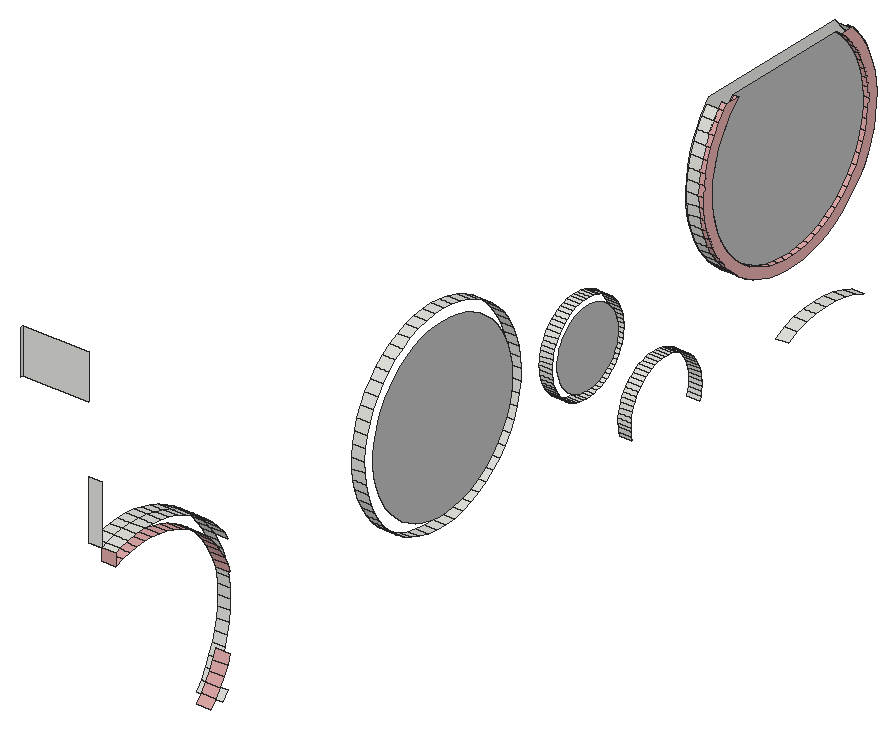
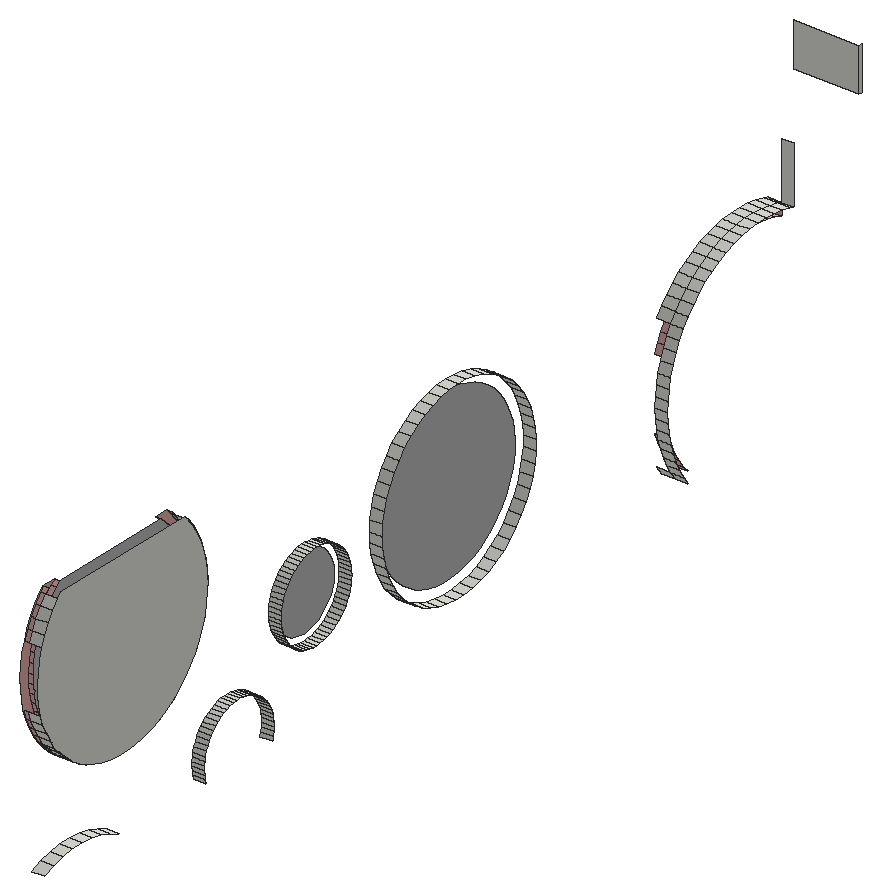
# SketchUp Ruby script. Lengths in inches.
U = 1.inch
M = Sketchup.active_model
def pt(a) = Geom::Point3d.new(a.map { |v| v * U })
def face(e, loops, mat)
  f = e.add_face(loops[0].map { |a| pt(a) })
  loops[1..].each { |l| e.add_face(l.map { |a| pt(a) }).erase! }
  f.material = f.back_material = mat if mat
  f
end
# faces: each face lists its corners as indices into pts; further lists are holes
def faces(e, pts, list, mat = nil) = list.each { |f| face(e, (f[0].is_a?(Array) ? f : [f]).map { |l| l.map { |i| pts[i] } }, mat) }
# xy, xz, yz: faces in a plane at the given z, y or x. An outline is a flat list of corners, or four numbers for a rectangle; further outlines are holes
def ring(l) = l.size == 4 ? [[l[0], l[1]], [l[2], l[1]], [l[2], l[3]], [l[0], l[3]]] : l.each_slice(2).to_a
def flat(e, list, mat, &to3) = list.each { |f| face(e, (f[0].is_a?(Array) ? f : [f]).map { |l| ring(l).map { |u, v| to3.(u, v) } }, mat) }
def xy(e, z, list, mat = nil) = flat(e, list, mat) { |x, y| [x, y, z] }
def xz(e, y, list, mat = nil) = flat(e, list, mat) { |x, z| [x, y, z] }
def yz(e, x, list, mat = nil) = flat(e, list, mat) { |y, z| [x, y, z] }
def lines(e, pts, list) = list.each { |a, b| e.add_line(pt(pts[a]), pt(pts[b])) }
# prism: a flat outline (further loops are holes) pulled along v
def prism(e, loops, v, mat = nil)
  f = face(e, loops, mat); d = Geom::Vector3d.new(v.map { |x| x * U })
  f.pushpull(f.normal.samedirection?(d) ? d.length : -d.length)
end
def box(e, o, s, mat = nil) = prism(e, [[o, [o[0] + s[0], o[1], o[2]], [o[0] + s[0], o[1] + s[1], o[2]], [o[0], o[1] + s[1], o[2]]]], [0, 0, s[2]], mat)
def at(x, y, z, deg = 0) = Geom::Transformation.translation(pt([x, y, z])) * Geom::Transformation.rotation(ORIGIN, Z_AXIS, deg.degrees)
def axes(o, x, y, z) = Geom::Transformation.new([*x, 0, *y, 0, *z, 0, *pt(o).to_a, 1])
def part(name) = M.definitions.add(name)
# library, detail: a bought-in or finely detailed component or shape, given as its bounding box
def library(name, o, s) = part(name).tap { |d| box(d.entities, o, s) }
def detail(e, o, s) = box(e.add_group.entities, o, s)
def put(e, d, t, mat = nil) = e.add_instance(d, t).tap { |i| i.material = mat if mat }
def group(e, t, mat = nil) = e.add_group.tap { |g| g.transformation = t; g.material = mat if mat }.entities
root = M.entities
M.materials.add("Generic").color = [224, 169, 169]
M.materials.add("[Mirror 01]").color = [185, 185, 185]
xy(root,95.3,[[9,116.01,10.6875,117.43]])
xy(root,95.3,[[10.6875,116.01,11.4375,117.43]],"Generic")
xy(root,96.65,[[10.6875,116.08,11.4375,117.37]],"Generic")
xz(root,0.4375,[[9,112.04,10.6875,120],[0,129.25,9,135.25]])
xz(root,0.4375,[[10.6875,110.34,12.625,112.04]],"Generic")
xz(root,89.3,[[9,99.77,10.6875,100.36]])
xz(root,102.58,[[9,86.91,10.6875,87.49]])
yz(root,0,[[0,129.25,0.4375,135.25]])
yz(root,9,[[116.01,95.3,117.43,95.3,118.85,95.43,120.24,95.71,121.6,96.11,122.91,96.65,124.17,97.31,125.36,98.09,126.46,98.97,127.48,99.97,128.4,101.05,129.2,102.22,129.89,103.46,130.46,104.76,130.9,106.11,131.2,107.5,131.375,108.91,131.41,110.32,131.31,111.74,131.07,113.14,130.69,114.51,130.19,115.84,129.5625,117.11,128.8125,118.3125,127.95,119.44,127.43,120,106.01,120,105.5,119.44,104.63,118.3125,103.89,117.11,103.26,115.84,102.75,114.51,102.38,113.14,102.14,111.74,102.04,110.32,102.07,108.91,102.24,107.5,102.55,106.11,102.99,104.76,103.56,103.46,104.25,102.22,105.05,101.05,105.97,99.97,106.98,98.97,108.09,98.09,109.28,97.31,110.53,96.65,111.85,96.11,113.21,95.71,114.6,95.43]])
yz(root,10.6875,[[59,90.55,60.3,90.67,61.57,90.94,62.81,91.35,63.99,91.89,65.11,92.55,66.15,93.34,67.09,94.23,67.93,95.23,68.66,96.31,69.26,97.46,69.73,98.67,70.07,99.93,70.27,101.22,70.32,102.52,70.23,103.81,70,105.1,69.625,106.34,69.12,107.54,68.48,108.68,67.73,109.74,66.86,110.7,65.89,111.57,64.83,112.33,63.69,112.96,62.49,113.47,61.25,113.84,59.96,114.07,58.67,114.16,57.37,114.11,56.08,113.91,54.82,113.57,53.61,113.1,52.46,112.49,51.38,111.77,50.39,110.93,49.49,109.98,48.71,108.94,48.04,107.82,47.5,106.64,47.1,105.4,46.83,104.13,46.71,102.83,46.72,101.53,46.89,100.24,47.1875,98.97,47.63,97.75,48.2,96.58,48.9,95.48,49.71,94.47,50.63,93.55,51.65,92.73,52.75,92.04,53.92,91.47,55.14,91.03,56.41,90.72,57.7,90.5625],[83.1,94.84,83.6,94.86,84.1,94.92,84.59,95.03,85.07,95.19,85.52,95.39,85.96,95.64,86.37,95.93,86.75,96.25,87.1,96.61,87.41,97.01,87.69,97.43,87.92,97.87,88.1,98.34,88.24,98.82,88.34,99.31,88.38,99.81,88.38,100.3125,88.33,100.81,88.23,101.3,88.08,101.78,87.89,102.24,87.66,102.6875,87.38,103.1,87.0625,103.49,86.71,103.85,86.33,104.17,85.91,104.45,85.47,104.69,85.01,104.89,84.53,105.04,84.04,105.15,83.55,105.21,83.04,105.22,82.55,105.18,82.05,105.09,81.57,104.96,81.1,104.78,80.65,104.55,80.23,104.28,79.83,103.98,79.47,103.63,79.14,103.26,78.84,102.85,78.59,102.42,78.38,101.96,78.22,101.49,78.1,101,78.03,100.5,78.01,100,78.04,99.5,78.11,99.01,78.24,98.52,78.41,98.05,78.62,97.6,78.875,97.16,79.17,96.76,79.51,96.39,79.875,96.05,80.28,95.75,80.7,95.48,81.15,95.26,81.625,95.09,82.11,94.96,82.6,94.88],[116.08,96.65,117.37,96.65,118.65,96.78,119.91,97.03,121.15,97.39,122.34,97.88,123.48,98.48,124.56,99.18,125.5625,99.99,126.49,100.89,127.32,101.875,128.05,102.9375,128.67,104.0625,129.1875,105.24,129.59,106.47,129.86,107.73,130.02,109,130.05,110.29,129.96,111.58,129.74,112.85,129.4,114.09,128.94,115.29,128.375,116.45,127.69,117.54,126.91,118.57,126.04,119.51,125.48,120,107.97,120,107.41,119.51,106.53,118.57,105.75,117.54,105.07,116.45,104.5,115.29,104.04,114.09,103.71,112.85,103.49,111.58,103.4,110.29,103.43,109,103.58,107.73,103.86,106.47,104.26,105.24,104.77,104.0625,105.4,102.94,106.13,101.875,106.96,100.89,107.88,99.99,108.89,99.18,109.97,98.48,111.11,97.88,112.3,97.39,113.53,97.03,114.8,96.78]],"[Mirror 01]")
yz(root,11.4375,[[116.01,95.3,117.43,95.3,118.85,95.43,120.24,95.71,121.6,96.11,122.91,96.65,124.17,97.31,125.36,98.09,126.46,98.97,127.48,99.97,128.4,101.05,129.2,102.22,129.89,103.46,130.46,104.76,130.9,106.11,131.2,107.5,131.375,108.91,131.41,110.32,131.31,111.74,131.07,113.14,130.69,114.51,130.19,115.84,129.5625,117.11,128.8125,118.3125,127.95,119.44,127.43,120,125.48,120,126.04,119.51,126.91,118.57,127.69,117.54,128.375,116.45,128.94,115.29,129.4,114.09,129.74,112.85,129.96,111.58,130.05,110.29,130.02,109,129.86,107.73,129.59,106.47,129.1875,105.24,128.67,104.0625,128.05,102.9375,127.32,101.875,126.49,100.89,125.5625,99.99,124.56,99.18,123.48,98.48,122.34,97.88,121.15,97.39,119.91,97.03,118.65,96.78,117.37,96.65,116.08,96.65,114.8,96.78,113.53,97.03,112.3,97.39,111.11,97.88,109.97,98.48,108.89,99.18,107.88,99.99,106.96,100.89,106.13,101.875,105.4,102.94,104.77,104.0625,104.26,105.24,103.86,106.47,103.58,107.73,103.43,109,103.4,110.29,103.49,111.58,103.71,112.85,104.04,114.09,104.5,115.29,105.07,116.45,105.75,117.54,106.53,118.57,107.41,119.51,107.97,120,106.01,120,105.5,119.44,104.63,118.3125,103.89,117.11,103.26,115.84,102.75,114.51,102.38,113.14,102.14,111.74,102.04,110.32,102.07,108.91,102.24,107.5,102.55,106.11,102.99,104.76,103.56,103.46,104.25,102.22,105.05,101.05,105.97,99.97,106.98,98.97,108.09,98.09,109.28,97.31,110.53,96.65,111.85,96.11,113.21,95.71,114.6,95.43]],"Generic")
p = [[10.6875,102.25,85.2],[10.6875,102.42,85.76],[9,102.42,85.76],[9,102.25,85.2],[10.6875,90.64,85.98],[10.6875,90.78,85.41],
  [9,90.78,85.41],[9,90.64,85.98],[10.6875,118.89,86.29],[10.6875,117.37,85.6],[9,117.37,85.6],[9,118.89,86.29],
  [10.6875,17.5,86.78],[10.6875,16.67,85.82],[12.625,16.67,85.82],[12.625,17.5,86.78],[10.6875,18.75,85.78],[10.6875,19.58,86.91],
  [9,19.58,86.91],[9,18.75,85.78],[12.625,19.58,86.91],[12.625,18.75,85.78],[10.6875,102.53,86.33],[9,102.53,86.33],
  [10.6875,90.55,86.55],[9,90.55,86.55],[10.6875,130.28,85.99],[10.6875,128.72,86.59],[9,128.72,86.59],[9,130.28,85.99],
  [10.6875,102.58,86.91],[9,102.58,86.91],[10.6875,120.48,86.8125],[9,120.48,86.8125],[10.6875,90.52,87.13],[9,90.52,87.13],
  [10.6875,127.1,87.01],[9,127.1,87.01],[10.6875,18.24,87.8],[12.625,18.24,87.8],[10.6875,122.11,87.15],[9,122.11,87.15],
  [10.6875,20.3,88.11],[9,20.3,88.11],[10.6875,125.45,87.25],[9,125.45,87.25],[10.6875,90.54,87.72],[9,90.54,87.72],
  [10.6875,123.78,87.29],[9,123.78,87.29],[10.6875,102.58,87.49],[10.6875,102.52,88.07],[9,102.52,88.07],[9,102.58,87.49],
  [10.6875,90.625,88.29],[9,90.625,88.29],[10.6875,18.9,88.88],[12.625,18.9,88.88],[10.6875,20.92,89.36],[9,20.92,89.36],
  [10.6875,102.4,88.64],[9,102.4,88.64],[10.6875,90.76,88.86],[9,90.76,88.86],[10.6875,102.23,89.2],[9,102.23,89.2],
  [10.6875,19.46,90.01],[12.625,19.46,90.01],[10.6875,90.95,89.41],[9,90.95,89.41],[10.6875,56.14,89.23],[10.6875,57.6,89.04],
  [9,57.6,89.04],[9,56.14,89.23],[10.6875,59.06,89.02],[9,59.06,89.02],[10.6875,60.53,89.17],[9,60.53,89.17],
  [10.6875,54.71,89.57],[9,54.71,89.57],[10.6875,61.96,89.47],[9,61.96,89.47],[10.6875,102.01,89.74],[9,102.01,89.74],
  [10.6875,21.44,90.66],[9,21.44,90.66],[10.6875,91.19,89.94],[9,91.19,89.94],[10.6875,63.36,89.93],[9,63.36,89.93],
  [10.6875,53.32,90.0625],[9,53.32,90.0625],[10.6875,101.73,90.26],[9,101.73,90.26],[10.6875,64.7,90.54],[9,64.7,90.54],
  [10.6875,91.49,90.45],[9,91.49,90.45],[10.6875,19.92,91.19],[12.625,19.92,91.19],[10.6875,52,90.71],[9,52,90.71],
  [10.6875,101.41,90.74],[9,101.41,90.74],[10.6875,91.83,90.92],[9,91.83,90.92],[10.6875,65.96,91.29],[9,65.96,91.29],
  [10.6875,21.84,92],[9,21.84,92],[10.6875,50.76,91.49],[9,50.76,91.49],[10.6875,101.04,91.19],[9,101.04,91.19],
  [10.6875,92.21,91.36],[9,92.21,91.36],[10.6875,100.64,91.61],[9,100.64,91.61],[10.6875,67.13,92.18],[9,67.13,92.18],
  [10.6875,92.63,91.76],[9,92.63,91.76],[10.6875,49.62,92.41],[9,49.62,92.41],[10.6875,100.1875,91.98],[9,100.1875,91.98],
  [10.6875,93.1,92.11],[9,93.1,92.11],[10.6875,22.14,93.37],[9,22.14,93.37],[10.6875,99.71,92.3125],[9,99.71,92.3125],
  [10.6875,93.59,92.42],[9,93.59,92.42],[10.6875,68.2,93.1875],[9,68.2,93.1875],[10.6875,99.19,92.59],[9,99.19,92.59],
  [10.6875,48.58,93.45],[9,48.58,93.45],[10.6875,94.11,92.6875],[9,94.11,92.6875],[10.6875,98.66,92.82],[9,98.66,92.82],
  [10.6875,94.65,92.9],[9,94.65,92.9],[10.6875,98.1,93],[9,98.1,93],[10.6875,95.22,93.05],[9,95.22,93.05],
  [10.6875,97.53,93.12],[9,97.53,93.12],[10.6875,95.79,93.15],[9,95.79,93.15],[10.6875,96.95,93.1875],[9,96.95,93.1875],
  [10.6875,69.15,94.31],[9,69.15,94.31],[10.6875,96.37,93.2],[9,96.37,93.2],[10.6875,22.3125,94.76],[9,22.3125,94.76],
  [10.6875,47.66,94.6],[9,47.66,94.6],[10.6875,82.5,93.97],[10.6875,83.09,93.93],[9,83.09,93.93],[9,82.5,93.97],
  [10.6875,83.68,93.94],[9,83.68,93.94],[10.6875,84.26,94.02],[9,84.26,94.02],[10.6875,81.91,94.0625],[9,81.91,94.0625],
  [10.6875,84.84,94.15],[9,84.84,94.15],[10.6875,81.34,94.21],[9,81.34,94.21],[10.6875,85.4,94.33],[9,85.4,94.33],
  [10.6875,80.79,94.42],[9,80.79,94.42],[10.6875,69.97,95.53],[9,69.97,95.53],[10.6875,85.9375,94.57],[9,85.9375,94.57],
  [10.6875,80.26,94.68],[9,80.26,94.68],[10.6875,46.87,95.84],[9,46.87,95.84],[10.6875,86.45,94.86],[9,86.45,94.86],
  [10.6875,79.76,94.99],[9,79.76,94.99],[10.6875,22.375,96.15],[9,22.375,96.15],[10.6875,86.93,95.2],[9,86.93,95.2],
  [10.6875,79.29,95.34],[9,79.29,95.34],[10.6875,87.38,95.58],[9,87.38,95.58],[10.6875,78.85,95.74],[9,78.85,95.74],
  [10.6875,114.6,95.43],[10.6875,116.01,95.3],[9,116.01,95.3],[9,114.6,95.43],[11.4375,116.01,95.3],[11.4375,114.6,95.43],
  [10.6875,117.43,95.3],[10.6875,118.85,95.43],[9,118.85,95.43],[9,117.43,95.3],[11.4375,118.85,95.43],[11.4375,117.43,95.3],
  [10.6875,113.21,95.71],[9,113.21,95.71],[11.4375,113.21,95.71],[10.6875,120.24,95.71],[9,120.24,95.71],[11.4375,120.24,95.71],
  [10.6875,70.65,96.83],[9,70.65,96.83],[10.6875,87.79,96.01],[9,87.79,96.01],[10.6875,78.46,96.18],[9,78.46,96.18],
  [10.6875,111.85,96.11],[9,111.85,96.11],[11.4375,111.85,96.11],[10.6875,121.6,96.11],[9,121.6,96.11],[11.4375,121.6,96.11],
  [10.6875,46.22,97.16],[9,46.22,97.16],[10.6875,88.16,96.47],[9,88.16,96.47],[10.6875,110.53,96.65],[9,110.53,96.65],
  [11.4375,110.53,96.65],[10.6875,122.91,96.65],[9,122.91,96.65],[11.4375,122.91,96.65],[10.6875,22.32,97.55],[9,22.32,97.55],
  [10.6875,78.11,96.66],[9,78.11,96.66],[10.6875,88.48,96.97],[9,88.48,96.97],[10.6875,109.28,97.31],[9,109.28,97.31],
  [11.4375,109.28,97.31],[10.6875,124.17,97.31],[9,124.17,97.31],[11.4375,124.17,97.31],[10.6875,77.81,97.16],[9,77.81,97.16],
  [10.6875,116.08,96.65],[10.6875,114.8,96.78],[11.4375,114.8,96.78],[11.4375,116.08,96.65],[10.6875,118.65,96.78],[10.6875,117.37,96.65],
  [11.4375,117.37,96.65],[11.4375,118.65,96.78],[10.6875,71.18,98.2],[9,71.18,98.2],[10.6875,113.53,97.03],[11.4375,113.53,97.03],
  [10.6875,119.91,97.03],[11.4375,119.91,97.03],[10.6875,88.75,97.49],[9,88.75,97.49],[10.6875,112.3,97.39],[11.4375,112.3,97.39],
  [10.6875,121.15,97.39],[11.4375,121.15,97.39],[10.6875,45.73,98.54],[9,45.73,98.54],[10.6875,77.56,97.7],[9,77.56,97.7],
  [10.6875,108.09,98.09],[9,108.09,98.09],[11.4375,108.09,98.09],[10.6875,125.36,98.09],[9,125.36,98.09],[11.4375,125.36,98.09],
  [10.6875,111.11,97.88],[11.4375,111.11,97.88],[10.6875,122.34,97.88],[11.4375,122.34,97.88],[10.6875,88.97,98.04],[9,88.97,98.04],
  [10.6875,22.14,98.94],[9,22.14,98.94],[10.6875,77.36,98.25],[9,77.36,98.25],[10.6875,109.97,98.48],[11.4375,109.97,98.48],
  [10.6875,123.48,98.48],[11.4375,123.48,98.48],[10.6875,89.14,98.6],[9,89.14,98.6],[10.6875,106.98,98.97],[9,106.98,98.97],
  [11.4375,106.98,98.97],[10.6875,126.46,98.97],[9,126.46,98.97],[11.4375,126.46,98.97],[10.6875,71.5625,99.62],[9,71.5625,99.62],
  [10.6875,77.21,98.82],[9,77.21,98.82],[10.6875,45.39,99.97],[9,45.39,99.97],[10.6875,108.89,99.18],[11.4375,108.89,99.18],
  [10.6875,124.56,99.18],[11.4375,124.56,99.18],[10.6875,89.25,99.18],[9,89.25,99.18],[10.6875,77.125,99.41],[9,77.125,99.41],
  [10.6875,21.85,100.31],[9,21.85,100.31],[10.6875,105.97,99.97],[9,105.97,99.97],[11.4375,105.97,99.97],[10.6875,127.48,99.97],
  [9,127.48,99.97],[11.4375,127.48,99.97],[10.6875,89.3,99.77],[9,89.3,99.77],[10.6875,107.88,99.99],[11.4375,107.88,99.99],
  [10.6875,125.5625,99.99],[11.4375,125.5625,99.99],[10.6875,77.09,100],[9,77.09,100],[10.6875,71.78,101.07],[9,71.78,101.07],
  [10.6875,45.2,101.43],[9,45.2,101.43],[10.6875,77.12,100.59],[9,77.12,100.59],[10.6875,105.05,101.05],[9,105.05,101.05],
  [11.4375,105.05,101.05],[10.6875,106.96,100.89],[11.4375,106.96,100.89],[10.6875,126.49,100.89],[11.4375,126.49,100.89],[10.6875,128.4,101.05],
  [9,128.4,101.05],[11.4375,128.4,101.05],[10.6875,21.45,101.65],[9,21.45,101.65],[10.6875,89.3,100.36],[10.6875,89.24,100.95],
  [9,89.24,100.95],[9,89.3,100.36],[10.6875,77.2,101.17],[9,77.2,101.17],[10.6875,89.12,101.53],[9,89.12,101.53],
  [10.6875,106.13,101.875],[11.4375,106.13,101.875],[10.6875,127.32,101.875],[11.4375,127.32,101.875],[10.6875,19.47,102.3],[10.6875,19.94,101.125],
  [12.625,19.94,101.125],[12.625,19.47,102.3],[10.6875,71.84,102.54],[9,71.84,102.54],[10.6875,104.25,102.22],[9,104.25,102.22],
  [11.4375,104.25,102.22],[10.6875,129.2,102.22],[9,129.2,102.22],[11.4375,129.2,102.22],[10.6875,77.34,101.74],[9,77.34,101.74],
  [10.6875,45.18,102.89],[9,45.18,102.89],[10.6875,88.95,102.09],[9,88.95,102.09],[10.6875,20.9375,102.95],[9,20.9375,102.95],
  [10.6875,77.53,102.3],[9,77.53,102.3],[10.6875,105.4,102.94],[11.4375,105.4,102.94],[10.6875,128.05,102.9375],[11.4375,128.05,102.9375],
  [10.6875,88.72,102.64],[9,88.72,102.64],[10.6875,103.56,103.46],[9,103.56,103.46],[11.4375,103.56,103.46],[10.6875,129.89,103.46],
  [9,129.89,103.46],[11.4375,129.89,103.46],[10.6875,18.91,103.44],[12.625,18.91,103.44],[10.6875,77.78,102.84],[9,77.78,102.84],
  [10.6875,71.74,104],[9,71.74,104],[10.6875,88.44,103.16],[9,88.44,103.16],[10.6875,78.07,103.35],[9,78.07,103.35],
  [10.6875,45.32,104.36],[9,45.32,104.36],[10.6875,104.77,104.0625],[11.4375,104.77,104.0625],[10.6875,128.67,104.0625],[11.4375,128.67,104.0625],
  [10.6875,20.32,104.21],[9,20.32,104.21],[10.6875,88.12,103.65],[9,88.12,103.65],[10.6875,78.42,103.83],[9,78.42,103.83],
  [10.6875,18.26,104.52],[12.625,18.26,104.52],[10.6875,102.99,104.76],[9,102.99,104.76],[11.4375,102.99,104.76],[10.6875,130.46,104.76],
  [9,130.46,104.76],[11.4375,130.46,104.76],[10.6875,87.75,104.11],[9,87.75,104.11],[10.6875,78.81,104.27],[9,78.81,104.27],
  [10.6875,71.48,105.45],[9,71.48,105.45],[10.6875,87.33,104.53],[9,87.33,104.53],[10.6875,104.26,105.24],[11.4375,104.26,105.24],
  [10.6875,129.1875,105.24],[11.4375,129.1875,105.24],[10.6875,19.6,105.4],[9,19.6,105.4],[10.6875,79.24,104.68],[9,79.24,104.68],
  [10.6875,45.625,105.8],[9,45.625,105.8],[10.6875,17.52,105.54],[12.625,17.52,105.54],[10.6875,86.88,104.9],[9,86.88,104.9],
  [10.6875,79.7,105.04],[9,79.7,105.04],[10.6875,102.55,106.11],[9,102.55,106.11],[11.4375,102.55,106.11],[10.6875,130.9,106.11],
  [9,130.9,106.11],[11.4375,130.9,106.11],[10.6875,86.39,105.24],[9,86.39,105.24],[10.6875,80.2,105.35],[9,80.2,105.35],
  [10.6875,85.875,105.52],[9,85.875,105.52],[10.6875,103.86,106.47],[11.4375,103.86,106.47],[10.6875,129.59,106.47],[11.4375,129.59,106.47],
  [10.6875,18.78,106.54],[9,18.78,106.54],[12.625,18.78,106.54],[12.625,19.6,105.4],[10.6875,71.06,106.86],[9,71.06,106.86],
  [10.6875,80.73,105.62],[9,80.73,105.62],[10.6875,16.69,106.5],[12.625,16.69,106.5],[10.6875,85.33,105.75],[9,85.33,105.75],
  [10.6875,81.28,105.83],[9,81.28,105.83],[10.6875,46.08,107.19],[9,46.08,107.19],[10.6875,81.85,105.99],[9,81.85,105.99],
  [10.6875,84.77,105.93],[9,84.77,105.93],[10.6875,84.19,106.06],[9,84.19,106.06],[10.6875,82.43,106.09],[9,82.43,106.09],
  [10.6875,83.02,106.13],[9,83.02,106.13],[10.6875,83.61,106.125],[9,83.61,106.125],[10.6875,102.24,107.5],[9,102.24,107.5],
  [11.4375,102.24,107.5],[10.6875,15.79,107.39],[12.625,15.79,107.39],[10.6875,17.86,107.6],[9,17.86,107.6],[12.625,17.86,107.6],
  [10.6875,103.58,107.73],[11.4375,103.58,107.73],[10.6875,129.86,107.73],[11.4375,129.86,107.73],[10.6875,70.49,108.21],[9,70.49,108.21],
  [10.6875,46.69,108.53],[9,46.69,108.53],[10.6875,14.82,108.2],[12.625,14.82,108.2],[10.6875,102.07,108.91],[9,102.07,108.91],
  [11.4375,102.07,108.91],[10.6875,16.87,108.58],[9,16.87,108.58],[12.625,16.87,108.58],[10.6875,103.43,109],[11.4375,103.43,109],
  [10.6875,130.02,109],[11.4375,130.02,109],[10.6875,13.78,108.92],[12.625,13.78,108.92],[10.6875,69.77,109.49],[9,69.77,109.49],
  [10.6875,47.44,109.79],[9,47.44,109.79],[10.6875,15.79,109.47],[9,15.79,109.47],[12.625,15.79,109.47],[10.6875,12.6875,109.56],
  [12.625,12.6875,109.56],[10.6875,102.04,110.32],[9,102.04,110.32],[11.4375,102.04,110.32],[10.6875,103.4,110.29],[11.4375,103.4,110.29],
  [10.6875,130.05,110.29],[11.4375,130.05,110.29],[10.6875,14.64,110.28],[9,14.64,110.28],[12.625,14.64,110.28],[10.6875,68.92,110.6875],
  [9,68.92,110.6875],[10.6875,11.54,110.1],[12.625,11.54,110.1],[10.6875,48.33,110.96],[9,48.33,110.96],[10.6875,10.36,110.54],
  [12.625,10.36,110.54],[10.6875,0.4375,110.34],[10.6875,1.63,110.75],[12.625,1.63,110.75],[12.625,0.4375,110.34],[10.6875,13.43,110.98],
  [9,13.43,110.98],[12.625,13.43,110.98],[10.6875,102.14,111.74],[9,102.14,111.74],[11.4375,102.14,111.74],[10.6875,103.49,111.58],
  [11.4375,103.49,111.58],[10.6875,129.96,111.58],[11.4375,129.96,111.58],[10.6875,9.14,110.89],[12.625,9.14,110.89],[10.6875,67.93,111.78],
  [9,67.93,111.78],[10.6875,2.86,111.04],[12.625,2.86,111.04],[10.6875,7.9,111.13],[12.625,7.9,111.13],[10.6875,4.11,111.22],
  [12.625,4.11,111.22],[10.6875,12.17,111.58],[9,12.17,111.58],[12.625,12.17,111.58],[10.6875,49.34,112.03],[9,49.34,112.03],
  [10.6875,6.64,111.26],[12.625,6.64,111.26],[10.6875,5.38,111.29],[12.625,5.38,111.29],[10.6875,10.86,112.07],[9,10.86,112.07],
  [12.625,10.86,112.07],[10.6875,103.71,112.85],[11.4375,103.71,112.85],[10.6875,129.74,112.85],[11.4375,129.74,112.85],[10.6875,102.38,113.14],
  [9,102.38,113.14],[11.4375,102.38,113.14],[10.6875,66.84,112.76],[9,66.84,112.76],[10.6875,1.18,112.3],[10.6875,0.4375,112.04],
  [9,0.4375,112.04],[9,1.18,112.3],[12.625,0.4375,112.04],[12.625,1.18,112.3],[10.6875,50.46,112.98],[9,50.46,112.98],
  [10.6875,9.51,112.45],[9,9.51,112.45],[12.625,9.51,112.45],[10.6875,2.57,112.62],[9,2.57,112.62],[12.625,2.57,112.62],
  [10.6875,8.14,112.71],[9,8.14,112.71],[12.625,8.14,112.71],[10.6875,3.95,112.82],[9,3.95,112.82],[12.625,3.95,112.82],
  [10.6875,6.75,112.87],[9,6.75,112.87],[12.625,6.75,112.87],[10.6875,5.35,112.9],[9,5.35,112.9],[12.625,5.35,112.9],
  [10.6875,65.64,113.62],[9,65.64,113.62],[10.6875,104.04,114.09],[11.4375,104.04,114.09],[10.6875,129.4,114.09],[11.4375,129.4,114.09],
  [10.6875,51.68,113.8],[9,51.68,113.8],[10.6875,102.75,114.51],[9,102.75,114.51],[11.4375,102.75,114.51],[10.6875,64.36,114.33],
  [9,64.36,114.33],[10.6875,52.98,114.48],[9,52.98,114.48],[10.6875,104.5,115.29],[11.4375,104.5,115.29],[10.6875,128.94,115.29],
  [11.4375,128.94,115.29],[10.6875,63.01,114.9],[9,63.01,114.9],[10.6875,54.35,115.02],[9,54.35,115.02],[10.6875,103.26,115.84],
  [9,103.26,115.84],[11.4375,103.26,115.84],[10.6875,130.69,114.51],[10.6875,130.19,115.84],[9,130.19,115.84],[9,130.69,114.51],
  [11.4375,130.19,115.84],[11.4375,130.69,114.51],[10.6875,61.6,115.32],[9,61.6,115.32],[10.6875,55.77,115.4],[9,55.77,115.4],
  [10.6875,60.15,115.58],[9,60.15,115.58],[10.6875,105.07,116.45],[11.4375,105.07,116.45],[10.6875,128.375,116.45],[11.4375,128.375,116.45],
  [10.6875,57.22,115.62],[9,57.22,115.62],[10.6875,58.6875,115.68],[9,58.6875,115.68],[10.6875,103.89,117.11],[9,103.89,117.11],
  [11.4375,103.89,117.11],[10.6875,129.5625,117.11],[9,129.5625,117.11],[11.4375,129.5625,117.11],[10.6875,105.75,117.54],[11.4375,105.75,117.54],
  [10.6875,127.69,117.54],[11.4375,127.69,117.54],[10.6875,104.63,118.3125],[9,104.63,118.3125],[11.4375,104.63,118.3125],[10.6875,128.8125,118.3125],
  [9,128.8125,118.3125],[11.4375,128.8125,118.3125],[10.6875,106.53,118.57],[11.4375,106.53,118.57],[10.6875,126.91,118.57],[11.4375,126.91,118.57],
  [10.6875,105.5,119.44],[9,105.5,119.44],[11.4375,105.5,119.44],[10.6875,127.95,119.44],[9,127.95,119.44],[11.4375,127.95,119.44],
  [10.6875,107.41,119.51],[11.4375,107.41,119.51],[10.6875,126.04,119.51],[11.4375,126.04,119.51],[10.6875,106.01,120],[11.4375,106.01,120],
  [10.6875,127.43,120],[11.4375,127.43,120],[10.6875,107.97,120],[11.4375,107.97,120],[10.6875,125.48,120],[11.4375,125.48,120]]
faces(root,p,[[0,1,2,3],[4,5,6,7],[8,9,10,11],[16,17,18,19],[16,17,20,21],[1,22,23,2],[24,4,7,25],[26,27,28,29],
  [22,30,31,23],[32,8,11,33],[34,24,25,35],[27,36,37,28],[40,32,33,41],[17,42,43,18],[36,44,45,37],[46,34,35,47],
  [48,40,41,49],[44,48,49,45],[50,51,52,53],[54,46,47,55],[42,58,59,43],[51,60,61,52],[62,54,55,63],[60,64,65,61],
  [68,62,63,69],[70,71,72,73],[71,74,75,72],[74,76,77,75],[78,70,73,79],[76,80,81,77],[64,82,83,65],[58,84,85,59],
  [86,68,69,87],[80,88,89,81],[90,78,79,91],[82,92,93,83],[88,94,95,89],[96,86,87,97],[100,90,91,101],[92,102,103,93],
  [104,96,97,105],[94,106,107,95],[84,108,109,85],[110,100,101,111],[102,112,113,103],[114,104,105,115],[112,116,117,113],[106,118,119,107],
  [120,114,115,121],[122,110,111,123],[116,124,125,117],[126,120,121,127],[108,128,129,109],[124,130,131,125],[132,126,127,133],[118,134,135,119],
  [130,136,137,131],[138,122,123,139],[140,132,133,141],[136,142,143,137],[144,140,141,145],[142,146,147,143],[148,144,145,149],[146,150,151,147],
  [152,148,149,153],[150,154,155,151],[134,156,157,135],[158,152,153,159],[154,158,159,155],[128,160,161,129],[162,138,139,163],[164,165,166,167],
  [165,168,169,166],[168,170,171,169],[172,164,167,173],[170,174,175,171],[176,172,173,177],[174,178,179,175],[180,176,177,181],[156,182,183,157],
  [178,184,185,179],[186,180,181,187],[188,162,163,189],[184,190,191,185],[192,186,187,193],[160,194,195,161],[190,196,197,191],[198,192,193,199],
  [196,200,201,197],[202,198,199,203],[204,205,206,207],[210,211,212,213],[216,204,207,217],[211,219,220,212],[182,222,223,183],[200,224,225,201],
  [226,202,203,227],[228,216,217,229],[219,231,232,220],[234,188,189,235],[224,236,237,225],[238,228,229,239],[231,241,242,232],[194,244,245,195],
  [246,226,227,247],[236,248,249,237],[250,238,239,251],[241,253,254,242],[256,246,247,257],[222,266,267,223],[248,272,273,249],[278,234,235,279],
  [280,256,257,281],[282,250,251,283],[253,285,286,254],[272,292,293,273],[244,294,295,245],[296,280,281,297],[292,302,303,293],[304,282,283,305],
  [285,307,308,286],[266,310,311,267],[312,296,297,313],[314,278,279,315],[302,320,321,303],[322,312,313,323],[294,324,325,295],[326,304,305,327],
  [307,329,330,308],[320,332,333,321],[338,322,323,339],[310,340,341,311],[342,314,315,343],[344,338,339,345],[346,326,327,347],[329,353,354,330],
  [324,356,357,325],[358,359,360,361],[362,344,345,363],[359,364,365,360],[340,374,375,341],[376,346,347,377],[353,379,380,354],[382,362,363,383],
  [384,342,343,385],[364,386,387,365],[356,388,389,357],[390,382,383,391],[386,396,397,387],[398,376,377,399],[379,401,402,380],[406,390,391,407],
  [374,408,409,375],[396,410,411,397],[412,406,407,413],[414,384,385,415],[388,420,421,389],[410,422,423,411],[424,412,413,425],[428,398,399,429],
  [401,431,432,402],[422,434,435,423],[436,424,425,437],[408,438,439,409],[434,440,441,435],[420,446,447,421],[448,436,437,449],[450,414,415,451],
  [440,454,455,441],[456,448,449,457],[458,428,429,459],[431,461,462,432],[454,464,465,455],[466,456,457,467],[464,468,469,465],[446,474,475,447],
  [446,474,476,477],[438,478,479,439],[480,466,467,481],[468,484,485,469],[486,480,481,487],[488,450,451,489],[490,486,487,491],[484,492,493,485],
  [492,494,495,493],[496,490,491,497],[498,496,497,499],[500,498,499,501],[494,500,501,495],[502,458,459,503],[474,507,508,475],[474,507,509,476],
  [478,514,515,479],[516,488,489,517],[520,502,503,521],[507,523,524,508],[507,523,525,509],[514,532,533,515],[534,516,517,535],[523,536,537,524],
  [523,536,538,525],[541,520,521,542],[536,548,549,537],[536,548,550,538],[532,551,552,533],[555,534,535,556],[548,563,564,549],[548,563,565,550],
  [566,541,542,567],[551,575,576,552],[563,583,584,564],[563,583,585,565],[586,555,556,587],[583,592,593,584],[583,592,594,585],[599,566,567,600],
  [575,602,603,576],[604,605,606,607],[604,605,608,609],[610,586,587,611],[592,612,613,593],[592,612,614,594],[615,604,607,616],[615,604,609,617],
  [612,618,619,613],[612,618,620,614],[621,615,616,622],[621,615,617,623],[618,624,625,619],[618,624,626,620],[627,621,622,628],[627,621,623,629],
  [602,630,631,603],[624,627,628,625],[624,627,629,626],[636,610,611,637],[638,599,600,639],[630,641,642,631],[643,636,637,644],[641,649,650,642],
  [651,643,644,652],[653,638,639,654],[656,657,658,659],[649,662,663,650],[664,651,652,665],[662,666,667,663],[672,664,665,673],[674,672,673,675],
  [666,674,675,667],[676,653,654,677],[657,679,680,658],[686,676,677,687],[679,689,690,680],[696,686,687,697],[689,699,700,690]])
faces(root,p,[[12,13,14,15],[38,12,15,39],[56,38,39,57],[66,56,57,67],[98,66,67,99],[204,205,208,209],[210,211,214,215],[216,204,209,218],
  [211,219,221,214],[228,216,218,230],[219,231,233,221],[238,228,230,240],[231,241,243,233],[250,238,240,252],[241,253,255,243],[258,259,260,261],
  [262,263,264,265],[259,268,269,260],[270,262,265,271],[268,274,275,269],[276,270,271,277],[282,250,252,284],[253,285,287,255],[274,288,289,275],
  [290,276,277,291],[288,298,299,289],[300,290,291,301],[304,282,284,306],[285,307,309,287],[298,316,317,299],[318,300,301,319],[326,304,306,328],
  [307,329,331,309],[316,334,335,317],[336,318,319,337],[346,326,328,348],[334,349,350,335],[351,336,337,352],[329,353,355,331],[349,366,367,350],
  [368,351,352,369],[370,371,372,373],[376,346,348,378],[353,379,381,355],[366,392,393,367],[394,368,369,395],[398,376,378,400],[379,401,403,381],
  [404,370,373,405],[392,416,417,393],[418,394,395,419],[426,404,405,427],[428,398,400,430],[401,431,433,403],[416,442,443,417],[444,418,419,445],
  [452,426,427,453],[458,428,430,460],[431,461,463,433],[442,470,471,443],[472,444,445,473],[482,452,453,483],[502,458,460,504],[505,482,483,506],
  [470,510,511,471],[512,472,473,513],[518,505,506,519],[520,502,504,522],[510,526,527,511],[528,512,513,529],[530,518,519,531],[539,530,531,540],
  [541,520,522,543],[526,544,545,527],[546,528,529,547],[553,539,540,554],[557,553,554,558],[559,560,561,562],[566,541,543,568],[544,569,570,545],
  [571,546,547,572],[573,557,558,574],[560,577,578,561],[579,573,574,580],[577,581,582,578],[588,579,580,589],[581,590,591,582],[590,588,589,591],
  [569,595,596,570],[597,571,572,598],[599,566,568,601],[595,632,633,596],[634,597,598,635],[638,599,601,640],[632,645,646,633],[647,634,635,648],
  [653,638,640,655],[656,657,660,661],[645,668,669,646],[670,647,648,671],[676,653,655,678],[657,679,681,660],[668,682,683,669],[684,670,671,685],
  [686,676,678,688],[679,689,691,681],[682,692,693,683],[694,684,685,695],[696,686,688,698],[689,699,701,691],[692,702,703,693],[704,694,695,705],
  [706,696,698,707],[699,708,709,701],[702,710,711,703],[712,704,705,713]],"Generic")
